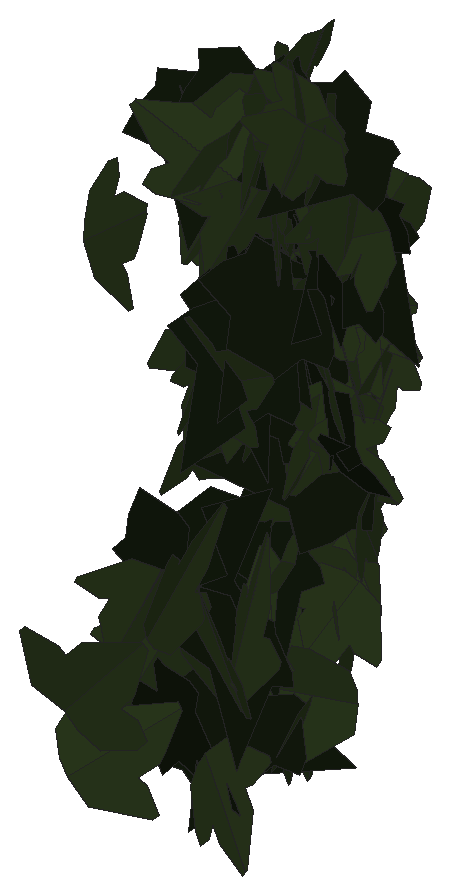
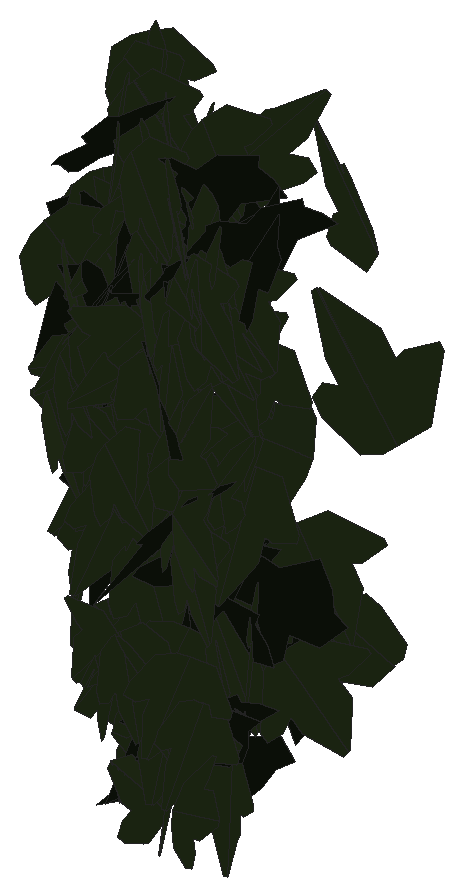
# SketchUp Ruby script. Lengths in inches.
U = 1.inch
M = Sketchup.active_model
def pt(a) = Geom::Point3d.new(a.map { |v| v * U })
def face(e, loops, mat)
  f = e.add_face(loops[0].map { |a| pt(a) })
  loops[1..].each { |l| e.add_face(l.map { |a| pt(a) }).erase! }
  f.material = f.back_material = mat if mat
  f
end
# faces: each face lists its corners as indices into pts; further lists are holes
def faces(e, pts, list, mat = nil) = list.each { |f| face(e, (f[0].is_a?(Array) ? f : [f]).map { |l| l.map { |i| pts[i] } }, mat) }
# xy, xz, yz: faces in a plane at the given z, y or x. An outline is a flat list of corners, or four numbers for a rectangle; further outlines are holes
def ring(l) = l.size == 4 ? [[l[0], l[1]], [l[2], l[1]], [l[2], l[3]], [l[0], l[3]]] : l.each_slice(2).to_a
def flat(e, list, mat, &to3) = list.each { |f| face(e, (f[0].is_a?(Array) ? f : [f]).map { |l| ring(l).map { |u, v| to3.(u, v) } }, mat) }
def xy(e, z, list, mat = nil) = flat(e, list, mat) { |x, y| [x, y, z] }
def xz(e, y, list, mat = nil) = flat(e, list, mat) { |x, z| [x, y, z] }
def yz(e, x, list, mat = nil) = flat(e, list, mat) { |y, z| [x, y, z] }
def lines(e, pts, list) = list.each { |a, b| e.add_line(pt(pts[a]), pt(pts[b])) }
# prism: a flat outline (further loops are holes) pulled along v
def prism(e, loops, v, mat = nil)
  f = face(e, loops, mat); d = Geom::Vector3d.new(v.map { |x| x * U })
  f.pushpull(f.normal.samedirection?(d) ? d.length : -d.length)
end
def box(e, o, s, mat = nil) = prism(e, [[o, [o[0] + s[0], o[1], o[2]], [o[0] + s[0], o[1] + s[1], o[2]], [o[0], o[1] + s[1], o[2]]]], [0, 0, s[2]], mat)
def at(x, y, z, deg = 0) = Geom::Transformation.translation(pt([x, y, z])) * Geom::Transformation.rotation(ORIGIN, Z_AXIS, deg.degrees)
def axes(o, x, y, z) = Geom::Transformation.new([*x, 0, *y, 0, *z, 0, *pt(o).to_a, 1])
def part(name) = M.definitions.add(name)
# library, detail: a bought-in or finely detailed component or shape, given as its bounding box
def library(name, o, s) = part(name).tap { |d| box(d.entities, o, s) }
def detail(e, o, s) = box(e.add_group.entities, o, s)
def put(e, d, t, mat = nil) = e.add_instance(d, t).tap { |i| i.material = mat if mat }
def group(e, t, mat = nil) = e.add_group.tap { |g| g.transformation = t; g.material = mat if mat }.entities
root = M.entities
M.materials.add("efeu1").color = [18, 25, 13]
M.materials.add("efeu2").color = [43, 57, 29]
c1 = part("ivyleaf_9")
p = [[1.54,2.16,1.25],[1.36,2.04,1.19],[-0.21,0.99,0.68],[-0.71,1.11,0.82],[-0.85,0.86,0.67],[-0.8,0.17,0.21],
  [-0.9,-0.01,0.1],[-0.67,-0.16,-0.02],[-0.08,-0.08,-0.05],[-0.03,-0.6,-0.4],[0.65,-0.88,-0.66],[0.83,-0.6,-0.49],
  [1.29,-0.42,-0.43],[1.8125,-0.07,-0.26],[1.21,0.44,0.15]]
faces(c1.entities,p,[[0,1,2,3,4,5,6,7,8,9,10,11,12,13,14]],"efeu1")
c2 = part("ivyleaf_10")
p = [[0,0.5,-0.03],[-0.0625,2.02,-0.43],[-0.19,2.01,-0.46],[-0.54,1.05,-0.29],[-0.52,0.625,-0.18],[-0.83,0.76,-0.28],
  [-1.16,0.64,-0.33],[-1.15,0.33,-0.24],[-0.77,-0.39,0.02],[-0.3,-0.51,0.16],[0.04,-0.48,0.23],[-0.02,2.01,-0.4375],
  [-0.06,2.01,-0.43],[0.04,-0.49,0.23],[0.67,-0.49,0.14],[1.38,0.36,-0.2],[1.375,0.51,-0.24],[0.81,0.65,-0.19],
  [0.62,0.59,-0.15],[0.6,1.09,-0.28],[0.5,1.23,-0.31]]
faces(c2.entities,p,[[0,1,2,3,4,5,6,7,8,9,10],[11,12,0,13,14,15,16,17,18,19,20]],"efeu2")
put(root,c1,axes([516.07,135.85,182.4375],[-0.31431,-0.69548,-0.14444],[0.06471,0.12925,-0.76319],[0.70737,-0.32085,0.00564]))
put(root,c2,axes([516.41,135.89,181.1],[-0.26681,-0.58561,0.33355],[-0.11217,-0.31514,-0.64303],[0.66454,-0.28832,0.02538]))
put(root,c2,axes([516.1,137.3125,172.98],[0.04989,-0.32848,0.58836],[0.28354,-0.52497,-0.31713],[0.61129,0.27031,0.09908]))
put(root,c2,axes([516.48,134.24,173.87],[-0.35329,-0.5784,0.42474],[-0.10082,-0.42872,-0.66768],[0.71048,-0.34845,0.11646]))
put(root,c2,axes([516.3,137.07,177.6875],[0.23806,-0.54052,0.34973],[0.13751,-0.32157,-0.59061],[0.62893,0.2749,-0.00324]))
put(root,c1,axes([515.92,135.84,181.5],[0.10933,-0.25705,0.78758],[0.26806,-0.7407,-0.27896],[0.7839,0.28914,-0.01445]))
put(root,c2,axes([516.86,136.375,181.29],[-0.53452,-0.06601,0.52385],[-0.51044,-0.12602,-0.53672],[0.13502,-0.73774,0.0448]))
put(root,c2,axes([516.44,136.625,174.08],[-0.20093,-0.51899,-0.34534],[0.11795,0.32463,-0.5565],[0.61213,-0.23291,-0.00613]))
put(root,c2,axes([516.5,136.74,176.97],[0.13406,-0.68369,0.04869],[0.00227,-0.04917,-0.69667],[0.68542,0.13388,-0.00722]))
put(root,c2,axes([516.74,136.71,178.71],[-0.56427,0.28334,-0.29229],[-0.26427,0.12503,0.63139],[0.30964,0.62306,0.00622]))
put(root,c2,axes([516.625,136.07,180.67],[-0.09315,-0.66189,0.35511],[-0.04389,-0.35242,-0.6684],[0.74985,-0.10285,0.00499]))
put(root,c2,axes([516.77,135.51,172.45],[-0.5762,0.18721,0.25815],[-0.24323,0.08676,-0.60581],[-0.20622,-0.6254,-0.00677]))
put(root,c2,axes([516.02,133.27,181.29],[0.43527,-0.32687,-0.74749],[0.57456,-0.47865,0.54389],[-0.57919,-0.72048,-0.0222]))
put(root,c2,axes([516.66,135.05,177.25],[-0.13829,-0.67568,-0.46651],[0.07106,0.46146,-0.68942],[0.818,-0.15431,-0.01898]))
put(root,c2,axes([516.69,135.8125,181.59],[0.48048,-0.5197,-0.19845],[-0.0886,0.18738,-0.70524],[0.5492,0.48491,0.05984]))
put(root,c2,axes([516.62,136.17,177.54],[-0.08622,0.36395,0.64719],[0.17911,-0.6221,0.37371],[0.72058,0.19818,-0.01545]))
put(root,c2,axes([516.66,136.02,181.55],[-0.02214,-0.58779,0.48181],[0.20427,-0.46888,-0.56263],[0.73206,0.11305,0.17156]))
put(root,c2,axes([517.02,133.26,175.41],[-0.48479,-0.55595,0.32133],[-0.21596,-0.23802,-0.73761],[0.60473,-0.53068,-0.00581]))
put(root,c2,axes([516.8125,135.41,174.84],[0.13179,-0.77373,0.16641],[0.02695,-0.16421,-0.78487],[0.79096,0.13451,-0.00099]))
put(root,c2,axes([516.86,135.73,180.11],[0.76946,-0.08721,-0.22454],[-0.22349,0.02198,-0.77438],[0.08988,0.80126,-0.00319]))
put(root,c1,axes([516.43,134.53,174.82],[-0.26715,0.05858,0.77802],[0.73854,-0.24621,0.27213],[0.2516,0.7849,0.02729]))
put(root,c2,axes([516.92,134.4,174.96],[0.17626,-0.65964,-0.42013],[0.01313,0.43311,-0.6745],[0.78196,0.14142,0.10602]))
put(root,c2,axes([516.72,136.03,182.4],[-0.51602,0.38124,-0.31785],[0.19104,-0.27064,-0.63475],[-0.45812,-0.54227,0.09333]))
put(root,c2,axes([516.8125,136.54,174.72],[-0.44679,-0.41996,-0.24115],[0.19819,0.1408,-0.6124],[0.44186,-0.4878,0.03084]))
put(root,c1,axes([517.25,136.28,179.13],[-0.08595,0.32364,0.72585],[-0.16982,0.70574,-0.33479],[-0.77638,-0.1902,-0.00713]))
put(root,c2,axes([516.73,137.09,178.61],[-0.01863,-0.06959,0.70337],[0.34566,-0.61463,-0.05166],[0.61652,0.3425,0.05022]))
put(root,c2,axes([517.15,136.62,179.9],[-0.48332,-0.48124,0.19716],[-0.11158,-0.16693,-0.68099],[0.50795,-0.49457,0.03801]))
put(root,c2,axes([517.2,136.32,182.97],[0.31718,-0.465,-0.45066],[-0.25147,0.37398,-0.56287],[0.59673,0.40476,0.00234]))
put(root,c1,axes([516.67,136.46,177.65],[0.40102,-0.45053,-0.46464],[-0.09985,0.49699,-0.56808],[0.63945,0.36015,0.20268]))
put(root,c2,axes([517.06,136.35,180.4375],[0.05542,-0.61187,-0.33958],[0.00045,0.34067,-0.61377],[0.69979,0.04824,0.02729]))
put(root,c2,axes([517.28,134.4375,182.46],[0.2653,0.5468,0.55529],[-0.26224,-0.48974,0.60754],[0.73387,-0.37267,0.01636]))
put(root,c2,axes([517.01,134.5,179.17],[-0.59926,-0.32781,-0.19698],[0.18403,0.07381,-0.68269],[0.33525,-0.62647,0.02264]))
put(root,c1,axes([516.91,136.01,183.125],[-0.3707,-0.6188,-0.35039],[0.17413,0.30413,-0.72131],[0.68947,-0.40951,-0.00623]))
put(root,c1,axes([516.87,135.99,181.7],[-0.04412,-0.79522,-0.04255],[0.0098,0.04207,-0.79641],[0.7963,-0.04458,0.00744]))
put(root,c1,axes([517.03,136.06,173.59],[-0.29434,-0.71563,-0.02349],[0.00307,0.02413,-0.77377],[0.71601,-0.29428,-0.00633]))
put(root,c2,axes([517.1875,135.34,183.26],[-0.14952,-0.65758,0.24603],[0.03568,-0.25834,-0.6688],[0.70119,-0.12707,0.08649]))
put(root,c2,axes([517.22,136.97,183.4],[0.09325,-0.70303,0.1308],[-0.00247,-0.13222,-0.70892],[0.71509,0.09122,-0.0195]))
put(root,c2,axes([517.69,136.18,181.71],[-0.34214,0.0281,0.67312],[-0.67065,0.05762,-0.34329],[-0.0641,-0.75288,-0.00115]))
put(root,c2,axes([517.29,136.1,173.99],[-0.46433,-0.61169,-0.19589],[0.11687,0.15722,-0.76796],[0.63157,-0.4788,-0.00191]))
put(root,c1,axes([516.9,136.08,173.75],[0.02814,-0.46715,-0.61659],[0.20259,0.59991,-0.44527],[0.74657,-0.14518,0.14407]))
put(root,c2,axes([517.76,136.21,173.62],[0.16805,0.13555,-0.7043],[-0.70236,-0.11542,-0.1898],[-0.14527,0.71482,0.10291]))
put(root,c2,axes([517.4,134.57,182.72],[-0.05972,-0.75429,-0.11919],[-0.00216,0.11972,-0.75657],[0.76365,-0.05865,-0.01146]))
put(root,c2,axes([517.43,135.92,172.72],[-0.3696,0.47797,0.25833],[-0.18537,0.18275,-0.60335],[-0.51071,-0.41224,0.03205]))
put(root,c2,axes([517.28,136.05,174.83],[-0.58761,-0.30404,-0.24429],[0.21196,0.12187,-0.66153],[0.3274,-0.62459,-0.01016]))
put(root,c2,axes([517.04,135.24,178.34],[-0.34485,-0.23576,-0.59298],[0.56658,0.19698,-0.40782],[0.29358,-0.65707,0.0905]))
put(root,c2,axes([517.5,135.53,177.97],[0.1262,-0.5809,-0.46086],[-0.01435,0.46549,-0.59066],[0.74137,0.1079,0.06702]))
put(root,c1,axes([517.45,135.24,179.75],[-0.04903,-0.34116,0.7374],[0.33208,0.66581,0.33012],[-0.74153,0.32072,0.09908]))
put(root,c2,axes([517.4,134.24,179.16],[0.11074,-0.64099,0.29187],[0.12752,-0.27233,-0.64645],[0.69268,0.15261,0.07235]))
put(root,c2,axes([517.59,133.94,179.28],[0.14566,-0.65135,-0.4833],[-0.08368,0.47634,-0.6672],[0.80674,0.16701,0.01806]))
put(root,c2,axes([517.25,136.3,177.46],[-0.45591,0.42668,-0.33487],[0.26084,-0.21107,-0.62406],[-0.47555,-0.52482,-0.02127]))
put(root,c2,axes([517.52,135.85,173.86],[0.0769,-0.63436,0.29675],[0.01563,-0.29691,-0.63874],[0.70017,0.0763,-0.01833]))
put(root,c2,axes([517.46,136.4,180.93],[0.24502,-0.65295,0.10297],[0.06779,-0.08441,-0.69661],[0.65754,0.25202,0.03346]))
put(root,c2,axes([517.5,136.5,179.5],[-0.65113,-0.28772,0.04328],[0.03962,0.01742,0.71187],[-0.28824,0.65234,0.00007]))
put(root,c1,axes([517.21,135.29,176.04],[0.00793,-0.53012,-0.6409],[0.05937,0.63966,-0.52835],[0.82961,-0.04071,0.04393]))
put(root,c2,axes([517.74,134.76,181.75],[-0.38608,-0.51485,0.3183],[-0.17892,-0.2636,-0.64339],[0.57825,-0.42531,0.01345]))
put(root,c2,axes([517.59,136.88,175],[-0.07214,-0.67541,0.00443],[-0.00044,-0.00441,-0.67925],[0.67543,-0.07215,0.00003]))
put(root,c2,axes([518.07,135.97,182.3],[-0.07961,0.11088,-0.75229],[-0.59659,0.4599,0.13092],[0.4715,0.60064,0.03863]))
put(root,c2,axes([517.58,136.27,172.21],[0.20442,-0.52267,0.41884],[-0.11555,0.40382,0.56033],[-0.65974,-0.23267,0.03164]))
put(root,c2,axes([517.24,135.21,177.42],[0.16376,0.18074,-0.77114],[0.548,0.5427,0.24357],[0.57186,-0.5718,-0.01258]))
put(root,c1,axes([517.39,135.37,175.26],[-0.4465,-0.38149,-0.55998],[0.44389,0.34199,-0.58692],[0.51193,-0.62927,0.02051]))
put(root,c2,axes([517.75,136.16,181.09],[0.2261,-0.62599,-0.27759],[-0.06655,0.27086,-0.66502],[0.68154,0.23412,0.02716]))
put(root,c2,axes([517.09,131.71,173.02],[0.57614,-0.02285,-0.69861],[0.69886,0.03606,0.57517],[0.0133,-0.90482,0.04057]))
put(root,c1,axes([517.27,134.49,172.61],[0.31061,-0.12908,-0.7501],[0.07142,0.81153,-0.11007],[0.75777,-0.02358,0.31784]))
put(root,c2,axes([517.85,136.04,176.15],[-0.22337,-0.71318,0.13099],[-0.03076,-0.12762,-0.74729],[0.72446,-0.22531,0.00865]))
put(root,c2,axes([517.42,135.43,182.54],[0.04784,-0.16675,0.7924],[0.51841,-0.60348,-0.1583],[0.62206,0.51575,0.07098]))
put(root,c2,axes([517.9,135.5,179.84],[-0.11845,-0.66028,0.3021],[-0.04483,-0.29885,-0.67078],[0.72472,-0.1264,0.00788]))
put(root,c2,axes([517.85,136.79,178.13],[-0.04699,-0.63792,0.26533],[0.02081,-0.26713,-0.63856],[0.69058,-0.03536,0.03729]))
put(root,c1,axes([517.5625,134.74,180.28],[0.10408,-0.56039,-0.59148],[-0.08973,0.58477,-0.56983],[0.80984,0.13682,0.01288]))
put(root,c1,axes([517.24,133.2,173.54],[0.0181,-0.01786,-0.80652],[0.7753,0.22335,0.01245],[0.22296,-0.77519,0.02217]))
put(root,c1,axes([517.46,134.6875,179.45],[0.281,-0.79613,0.03812],[0.01321,-0.03576,-0.84426],[0.79693,0.28131,0.00055]))
put(root,c2,axes([517.82,135.91,179.62],[0.00404,0.08553,0.81445],[-0.00308,0.81446,-0.08551],[-0.81893,-0.00265,0.00434]))
put(root,c1,axes([518.32,135.83,178.07],[-0.281,-0.19036,0.68548],[-0.58946,-0.35034,-0.33893],[0.39832,-0.65276,-0.018]))
put(root,c2,axes([517.97,135.03,173.83],[0.39593,0.71423,-0.06043],[0.02253,0.0566,0.81659],[0.71643,-0.39649,0.00771]))
put(root,c2,axes([518.15,136.5,178.49],[-0.55677,-0.39305,0.14413],[-0.11477,-0.08733,-0.68151],[0.4026,-0.56846,0.00504]))
put(root,c2,axes([518.51,135.27,183.4],[-0.51298,-0.12537,0.52481],[-0.48733,-0.20321,-0.52489],[0.23163,-0.70518,0.05795]))
put(root,c2,axes([517.73,136.5625,180.29],[0.35463,0.36615,0.48682],[0.31038,0.37609,-0.50897],[-0.52414,0.47044,0.02799]))
put(root,c2,axes([518.2,136.61,180.25],[-0.30765,-0.53858,0.33019],[-0.02101,-0.35834,-0.60406],[0.63139,-0.27435,0.14079]))
put(root,c2,axes([518.01,135.6,175.14],[-0.18232,-0.42263,-0.67037],[0.30489,0.59753,-0.45963],[0.73147,-0.3544,0.02449]))
put(root,c1,axes([518.75,135.8125,176.9375],[-0.2601,-0.35452,-0.67933],[-0.39956,-0.5494,0.4397],[-0.65385,0.47676,0.00154]))
put(root,c2,axes([518.13,136.34,177.21],[-0.28284,-0.59362,-0.3974],[0.24658,0.32002,-0.65353],[0.67046,-0.36812,0.0727]))
put(root,c2,axes([517.9,135.15,181.82],[-0.18947,0.35478,-0.70623],[0.33293,-0.62283,-0.40221],[-0.71679,-0.38307,-0.00013]))
put(root,c2,axes([518.33,135.75,172.53],[0.08833,-0.66073,-0.05134],[0.00126,0.05197,-0.66655],[0.66272,0.08797,0.00811]))
put(root,c1,axes([518.3,134.33,173.35],[-0.37773,-0.71163,0.2055],[-0.07139,-0.19463,-0.8052],[0.73726,-0.38345,0.02732]))
put(root,c2,axes([517.88,136.84,175.09],[0.50979,0.06693,0.47907],[0.47844,0.03285,-0.5137],[-0.07132,0.69879,-0.02174]))
put(root,c2,axes([518.45,136.34,178.92],[0.65646,-0.03582,-0.25665],[-0.25353,0.05584,-0.65627],[0.05362,0.70263,0.03907]))
put(root,c2,axes([518.42,131.9,175.99],[0.21242,-0.57349,0.74298],[-0.26848,0.69281,0.61152],[-0.89934,-0.34228,-0.00707]))
put(root,c2,axes([518.9,134.96,183.54],[-0.39967,-0.02559,0.65672],[-0.63441,-0.18571,-0.39333],[0.17164,-0.74601,0.07539]))
put(root,c2,axes([517.97,135.64,182.69],[0.5605,-0.2042,0.53557],[0.49549,-0.20395,-0.59632],[0.28814,0.74793,-0.01638]))
put(root,c1,axes([518.72,135.57,177.5],[0.2266,-0.22521,0.70442],[-0.3848,0.59326,0.31346],[-0.63156,-0.44227,0.06176]))
put(root,c2,axes([519.01,135.13,173.25],[-0.03819,0.01051,-0.82546],[-0.81389,-0.13874,0.03589],[-0.13812,0.81461,0.01677]))
put(root,c2,axes([518.42,135.92,177.74],[0.07068,-0.50987,0.49944],[0.09199,-0.49119,-0.51447],[0.70777,0.11476,0.01699]))
put(root,c2,axes([518.55,135.07,172.91],[0.25284,-0.70242,-0.14184],[-0.04742,0.13368,-0.74654],[0.71503,0.25725,0.00064]))
put(root,c2,axes([518.75,132.98,174.33],[-0.7801,0.3793,-0.22604],[-0.20337,0.09867,0.86743],[0.39193,0.80617,0.00019]))
put(root,c1,axes([518.44,135.58,177.34],[0.66667,0.21685,-0.31888],[-0.3021,-0.10214,-0.70104],[-0.23968,0.73192,-0.00335]))
put(root,c1,axes([518.23,133.98,174.71],[0.02094,-0.78271,0.14834],[0.02326,-0.14772,-0.78276],[0.79631,0.02489,0.01897]))
put(root,c2,axes([518.63,135.99,173.98],[0.01323,0.0485,-0.70903],[-0.0733,0.70546,0.04689],[0.7069,0.07225,0.01813]))
put(root,c1,axes([518.74,135.82,181.64],[0.28997,0.457,-0.549],[-0.28325,-0.47037,-0.54116],[-0.65576,0.40525,-0.00901]))
put(root,c1,axes([518.49,134.03,179.82],[-0.34329,-0.71894,0.30983],[-0.09506,-0.29752,-0.79571],[0.77706,-0.35401,0.03953]))
put(root,c2,axes([518.7,135.88,177.95],[-0.37197,-0.52217,0.42701],[-0.10519,-0.43677,-0.62573],[0.66628,-0.36047,0.13961]))
put(root,c2,axes([518.48,137.1,179.62],[0.1435,-0.62167,0.28578],[0.13027,-0.26183,-0.63499],[0.67169,0.18359,0.0621]))
put(root,c2,axes([518.88,134.51,183.67],[0.17644,-0.33255,-0.74052],[-0.39241,0.62845,-0.37572],[0.71062,0.4296,-0.02362]))
put(root,c2,axes([518.51,135.63,181.5],[-0.06829,-0.37127,-0.64158],[0.23428,0.60046,-0.37242],[0.70326,-0.23608,0.06176]))
put(root,c2,axes([518.78,135.75,174.66],[0.68991,0.05647,-0.35141],[-0.34899,-0.04314,-0.6921],[-0.06987,0.77305,-0.01295]))
put(root,c2,axes([518.53,135.85,179.89],[0.00421,0.30158,0.77044],[0.03795,0.76956,-0.30145],[-0.82649,0.03687,-0.00991]))
put(root,c2,axes([518.77,135.54,178.23],[-0.64822,0.50048,0.01064],[0.00794,-0.00713,0.81894],[0.50053,0.64827,0.00079]))
put(root,c1,axes([518.26,136.46,180.72],[-0.20377,-0.328,-0.71954],[0.52274,0.50167,-0.37672],[0.59335,-0.55461,0.08478]))
put(root,c1,axes([518.67,135.65,180.74],[0.41597,-0.24378,-0.60507],[-0.49143,0.35481,-0.4808],[0.42899,0.64284,0.03592]))
put(root,c1,axes([518.67,134.59,180.55],[-0.36734,-0.70354,0.23615],[-0.05884,-0.23505,-0.79181],[0.73978,-0.36805,0.05428]))
put(root,c2,axes([518.24,133.35,179.3],[-0.51333,-0.02017,0.73254],[0.73153,-0.06717,0.51077],[0.04348,0.89197,0.05503]))
put(root,c2,axes([518.71,135.84,179.39],[-0.43932,0.63393,0.00103],[-0.00064,0.00081,-0.77128],[-0.63393,-0.43932,0.00006]))
put(root,c1,axes([518.65,136.28,180.34],[-0.18692,-0.53612,0.58713],[-0.06008,-0.59189,-0.5596],[0.79281,-0.17126,0.09602]))
put(root,c2,axes([518.55,135.625,177.37],[-0.4591,-0.31267,-0.53001],[0.46349,0.25928,-0.55443],[0.40478,-0.6515,0.03372]))
put(root,c2,axes([519.33,135.64,181.39],[0.43833,-0.10027,-0.70539],[-0.67253,0.2152,-0.4485],[0.23523,0.80212,0.03215]))
put(root,c1,axes([518.97,135.95,182.9],[-0.44251,-0.50001,0.42613],[-0.16837,-0.41031,-0.65629],[0.63502,-0.45722,0.12294]))
put(root,c2,axes([519.01,136.74,181.53],[-0.2881,-0.54663,0.41472],[-0.068,-0.42483,-0.6072],[0.68277,-0.27297,0.11451]))
put(root,c2,axes([519.16,134.31,183.58],[-0.64365,-0.20012,0.28154],[-0.24718,-0.14904,-0.67103],[0.24128,-0.68654,0.06361]))
put(root,c2,axes([518.93,136.84,178.625],[0.19808,-0.684,0.06765],[0.00432,-0.06916,-0.71194],[0.68732,0.19756,-0.01502]))
put(root,c2,axes([518.95,135.1,183.24],[0.21568,-0.58287,-0.42597],[0.01349,0.44775,-0.60584],[0.72181,0.1658,0.1386]))
put(root,c2,axes([518.98,136.42,181.11],[0.26535,-0.66463,-0.08562],[-0.02319,0.08293,-0.71558],[0.66972,0.2662,0.00915]))
put(root,c2,axes([518.76,136.63,178.68],[0.71999,-0.04013,0.1171],[0.11692,-0.0064,-0.72111],[0.04064,0.72943,0.00012]))
put(root,c2,axes([518.41,136.46,179.59],[0.27756,0.03968,0.66509],[0.64396,0.16892,-0.27882],[-0.17098,0.70061,0.02956]))
put(root,c2,axes([519.05,135.54,181.8],[-0.26371,-0.699,-0.02829],[0.00433,0.0286,-0.74707],[0.69956,-0.26368,-0.00604]))
put(root,c2,axes([518.9,132.51,172.97],[-0.06661,0.81263,0.14964],[-0.01073,0.14926,-0.81535],[-0.82622,-0.06746,-0.00147]))
put(root,c2,axes([518.58,129.48,175.56],[-0.78143,-0.19509,0.63211],[0.61733,0.13657,0.8053],[-0.23776,0.99577,0.01339]))
put(root,c2,axes([518.86,133.23,174.85],[0.78386,-0.56977,0.04211],[-0.03408,0.02474,0.96906],[-0.5703,-0.7846,-0.00002]))
put(root,c2,axes([519.2,135.82,176.15],[-0.12258,0.50345,0.43],[-0.32408,0.33572,-0.48545],[-0.57735,-0.29534,0.1812]))
